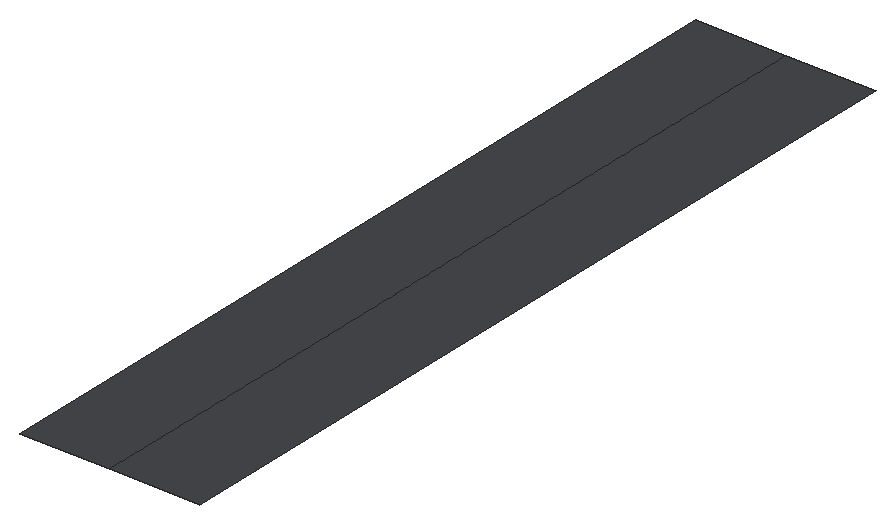
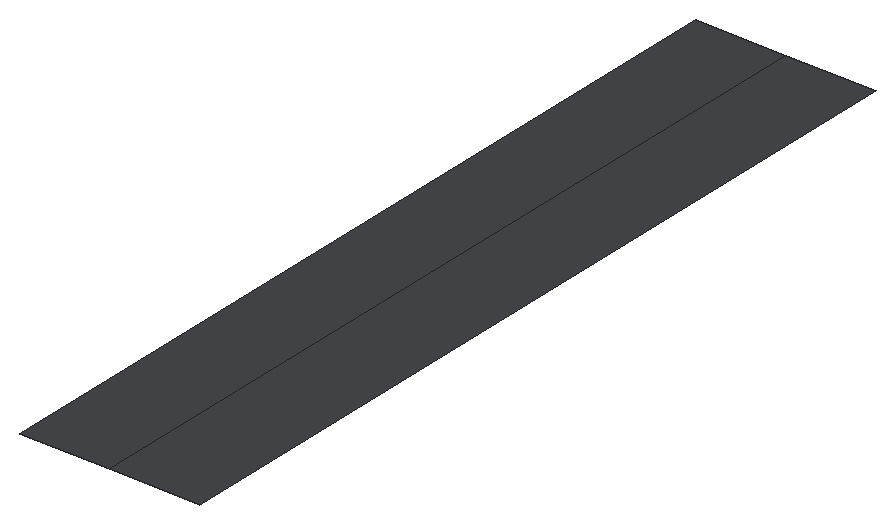
# SketchUp Ruby script. Lengths in inches.
U = 1.inch
M = Sketchup.active_model
def pt(a) = Geom::Point3d.new(a.map { |v| v * U })
def face(e, loops, mat)
  f = e.add_face(loops[0].map { |a| pt(a) })
  loops[1..].each { |l| e.add_face(l.map { |a| pt(a) }).erase! }
  f.material = f.back_material = mat if mat
  f
end
# faces: each face lists its corners as indices into pts; further lists are holes
def faces(e, pts, list, mat = nil) = list.each { |f| face(e, (f[0].is_a?(Array) ? f : [f]).map { |l| l.map { |i| pts[i] } }, mat) }
# xy, xz, yz: faces in a plane at the given z, y or x. An outline is a flat list of corners, or four numbers for a rectangle; further outlines are holes
def ring(l) = l.size == 4 ? [[l[0], l[1]], [l[2], l[1]], [l[2], l[3]], [l[0], l[3]]] : l.each_slice(2).to_a
def flat(e, list, mat, &to3) = list.each { |f| face(e, (f[0].is_a?(Array) ? f : [f]).map { |l| ring(l).map { |u, v| to3.(u, v) } }, mat) }
def xy(e, z, list, mat = nil) = flat(e, list, mat) { |x, y| [x, y, z] }
def xz(e, y, list, mat = nil) = flat(e, list, mat) { |x, z| [x, y, z] }
def yz(e, x, list, mat = nil) = flat(e, list, mat) { |y, z| [x, y, z] }
def lines(e, pts, list) = list.each { |a, b| e.add_line(pt(pts[a]), pt(pts[b])) }
# prism: a flat outline (further loops are holes) pulled along v
def prism(e, loops, v, mat = nil)
  f = face(e, loops, mat); d = Geom::Vector3d.new(v.map { |x| x * U })
  f.pushpull(f.normal.samedirection?(d) ? d.length : -d.length)
end
def box(e, o, s, mat = nil) = prism(e, [[o, [o[0] + s[0], o[1], o[2]], [o[0] + s[0], o[1] + s[1], o[2]], [o[0], o[1] + s[1], o[2]]]], [0, 0, s[2]], mat)
def at(x, y, z, deg = 0) = Geom::Transformation.translation(pt([x, y, z])) * Geom::Transformation.rotation(ORIGIN, Z_AXIS, deg.degrees)
def axes(o, x, y, z) = Geom::Transformation.new([*x, 0, *y, 0, *z, 0, *pt(o).to_a, 1])
def part(name) = M.definitions.add(name)
# library, detail: a bought-in or finely detailed component or shape, given as its bounding box
def library(name, o, s) = part(name).tap { |d| box(d.entities, o, s) }
def detail(e, o, s) = box(e.add_group.entities, o, s)
def put(e, d, t, mat = nil) = e.add_instance(d, t).tap { |i| i.material = mat if mat }
def group(e, t, mat = nil) = e.add_group.tap { |g| g.transformation = t; g.material = mat if mat }.entities
root = M.entities
M.materials.add("1432 AP 8245 TAR ROAD").color = [71, 72, 75]
M.materials.add("Outer Light").color = [251, 217, 152]
xy(root,171.29,[[278.68,95.37,278.84,96.87],[278.84,95.37,279,96.87]],"1432 AP 8245 TAR ROAD")
xy(root,171.29,[[278.68,95.37,278.84,96.87]],"Outer Light")
